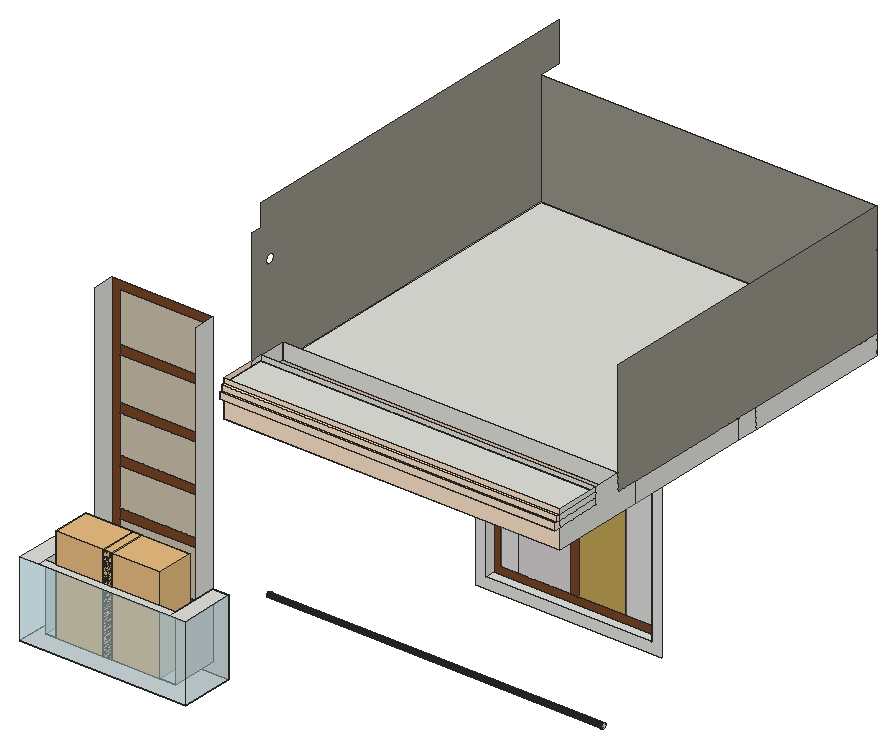
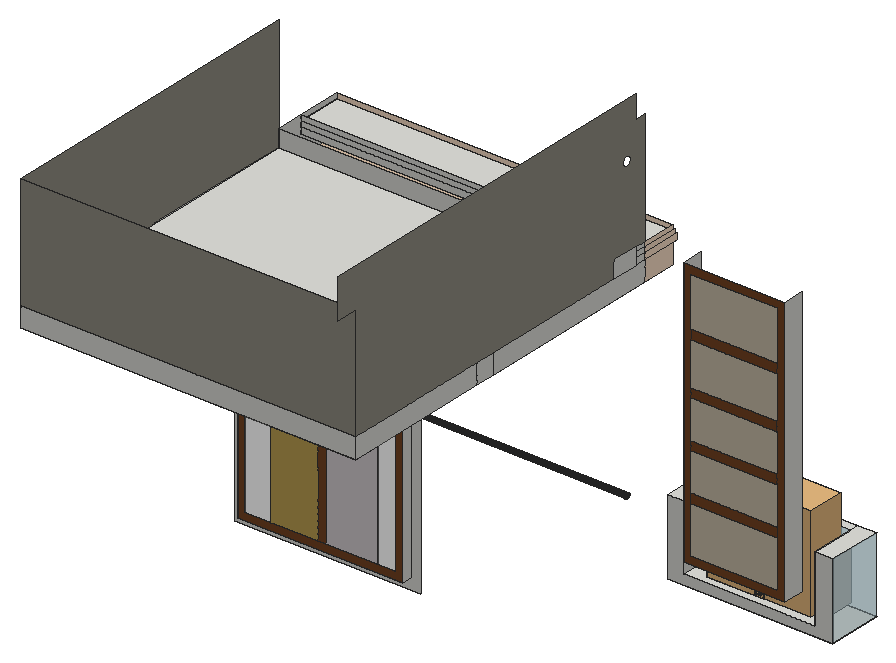
# SketchUp Ruby script. Lengths in inches.
U = 1.inch
M = Sketchup.active_model
def pt(a) = Geom::Point3d.new(a.map { |v| v * U })
def face(e, loops, mat)
  f = e.add_face(loops[0].map { |a| pt(a) })
  loops[1..].each { |l| e.add_face(l.map { |a| pt(a) }).erase! }
  f.material = f.back_material = mat if mat
  f
end
# faces: each face lists its corners as indices into pts; further lists are holes
def faces(e, pts, list, mat = nil) = list.each { |f| face(e, (f[0].is_a?(Array) ? f : [f]).map { |l| l.map { |i| pts[i] } }, mat) }
# xy, xz, yz: faces in a plane at the given z, y or x. An outline is a flat list of corners, or four numbers for a rectangle; further outlines are holes
def ring(l) = l.size == 4 ? [[l[0], l[1]], [l[2], l[1]], [l[2], l[3]], [l[0], l[3]]] : l.each_slice(2).to_a
def flat(e, list, mat, &to3) = list.each { |f| face(e, (f[0].is_a?(Array) ? f : [f]).map { |l| ring(l).map { |u, v| to3.(u, v) } }, mat) }
def xy(e, z, list, mat = nil) = flat(e, list, mat) { |x, y| [x, y, z] }
def xz(e, y, list, mat = nil) = flat(e, list, mat) { |x, z| [x, y, z] }
def yz(e, x, list, mat = nil) = flat(e, list, mat) { |y, z| [x, y, z] }
def lines(e, pts, list) = list.each { |a, b| e.add_line(pt(pts[a]), pt(pts[b])) }
# prism: a flat outline (further loops are holes) pulled along v
def prism(e, loops, v, mat = nil)
  f = face(e, loops, mat); d = Geom::Vector3d.new(v.map { |x| x * U })
  f.pushpull(f.normal.samedirection?(d) ? d.length : -d.length)
end
def box(e, o, s, mat = nil) = prism(e, [[o, [o[0] + s[0], o[1], o[2]], [o[0] + s[0], o[1] + s[1], o[2]], [o[0], o[1] + s[1], o[2]]]], [0, 0, s[2]], mat)
def at(x, y, z, deg = 0) = Geom::Transformation.translation(pt([x, y, z])) * Geom::Transformation.rotation(ORIGIN, Z_AXIS, deg.degrees)
def axes(o, x, y, z) = Geom::Transformation.new([*x, 0, *y, 0, *z, 0, *pt(o).to_a, 1])
def part(name) = M.definitions.add(name)
# library, detail: a bought-in or finely detailed component or shape, given as its bounding box
def library(name, o, s) = part(name).tap { |d| box(d.entities, o, s) }
def detail(e, o, s) = box(e.add_group.entities, o, s)
def put(e, d, t, mat = nil) = e.add_instance(d, t).tap { |i| i.material = mat if mat }
def group(e, t, mat = nil) = e.add_group.tap { |g| g.transformation = t; g.material = mat if mat }.entities
root = M.entities
M.materials.add("[Blinds Cellular White]1").color = [217, 211, 213]
M.materials.add("[Blinds Cloth Horizontal]").color = [192, 163, 85]
M.materials.add("[Color C01]").color = [255, 229, 204]
M.materials.add("[Formica Graystone]").color = [149, 146, 135]
M.materials.add("[Formica Laminate Dark]").color = [50, 53, 60]
M.materials.add("[Formica Laminate Light]").color = [213, 189, 164]
M.materials.add("[Siding Rusty Metal]").color = [206, 195, 174]
M.materials.add("[Translucent Glass Gray]").color = [128, 128, 128]
M.materials["[Translucent Glass Gray]"].alpha = 0.5
M.materials.add("[Translucent Glass Safety]").color = [204, 235, 244]
M.materials["[Translucent Glass Safety]"].alpha = 0.5
M.materials.add("[Wood Veneer 01]").color = [120, 70, 37]
c1 = library("Flora+17",[-57.52,158.6,-38.64],[66.99,62.88,77.28])
xy(root,1210.6875,[[114.55,552.4,668.12,733.78]])
xy(root,1243.125,[[176.52,580.17,613.71,733.78]])
xy(root,1330.35,[[218.87,733.78,559.3,805.03]])
xy(root,1365.38,[[1023.52,1367.21,1578.7,1398.39]])
xy(root,1460,[[1548.73,797.03,1550.53,797.27,1552.2,797.96,1553.64,799.06,1554.74,800.5,1555.43,802.17,1555.67,803.97,1555.43,805.77,1554.74,807.4375,1553.64,808.875,1552.2,809.98,1550.53,810.67,1548.73,810.91,1546.9375,810.67,1545.26,809.98,1543.83,808.875,1542.73,807.4375,1542.03,805.77,1541.8,803.97,1542.03,802.17,1542.73,800.5,1543.83,799.06,1545.26,797.96,1546.9375,797.27]])
xy(root,1460.3125,[[1828.92,797.03,1830.72,797.27,1832.39,797.96,1833.83,799.06,1834.93,800.5,1835.62,802.17,1835.86,803.97,1835.62,805.77,1834.93,807.4375,1833.83,808.875,1832.39,809.98,1830.72,810.67,1828.92,810.91,1827.125,810.67,1825.45,809.98,1824.02,808.875,1822.91,807.4375,1822.22,805.77,1821.98,803.97,1822.22,802.17,1822.91,800.5,1824.02,799.06,1825.45,797.96,1827.125,797.27]])
xy(root,1460.71,[[831.73,797.03,833.53,797.27,835.2,797.96,836.64,799.06,837.74,800.5,838.43,802.17,838.67,803.97,838.43,805.77,837.74,807.4375,836.64,808.875,835.2,809.98,833.53,810.67,832.41,810.82,831.05,810.82,829.9375,810.67,828.26,809.98,826.83,808.875,825.73,807.4375,825.03,805.77,824.8,803.97,825.03,802.17,825.73,800.5,826.83,799.06,828.26,797.96,829.9375,797.27],[831.05,810.82,832.41,810.82,831.73,810.91]])
xy(root,1460.9375,[[1269.3,797.03,1271.09,797.27,1272.76,797.96,1274.2,799.06,1275.3,800.5,1276,802.17,1276.23,803.97,1276,805.77,1275.3,807.4375,1274.2,808.875,1272.76,809.98,1271.09,810.67,1269.3,810.91,1267.5,810.67,1265.83,809.98,1264.39,808.875,1263.29,807.4375,1262.59,805.77,1262.36,803.97,1262.59,802.17,1263.29,800.5,1264.39,799.06,1265.83,797.96,1267.5,797.27]])
xy(root,1462.7,[[778.8,797.03,780.59,797.27,782.26,797.96,783.7,799.06,784.8,800.5,785.5,802.17,785.73,803.97,785.5,805.77,784.8,807.4375,783.7,808.875,782.26,809.98,780.59,810.67,778.8,810.91,777,810.67,775.33,809.98,773.89,808.875,772.79,807.4375,772.09,805.77,771.86,803.97,772.09,802.17,772.79,800.5,773.89,799.06,775.33,797.96,777,797.27],[893.3,797.03,895.09,797.27,896.76,797.96,898.2,799.06,899.3,800.5,900,802.17,900.23,803.97,900,805.77,899.3,807.4375,898.2,808.875,896.76,809.98,895.09,810.67,893.3,810.91,891.5,810.67,889.83,809.98,888.39,808.875,887.29,807.4375,886.59,805.77,886.36,803.97,886.59,802.17,887.29,800.5,888.39,799.06,889.83,797.96,891.5,797.27],[959.23,797.03,961.03,797.27,962.7,797.96,964.14,799.06,965.24,800.5,965.93,802.17,966.17,803.97,965.93,805.77,965.24,807.4375,964.14,808.875,962.7,809.98,961.03,810.67,959.23,810.91,957.4375,810.67,955.76,809.98,954.33,808.875,953.23,807.4375,952.53,805.77,952.3,803.97,952.53,802.17,953.23,800.5,954.33,799.06,955.76,797.96,957.4375,797.27],[1015.98,797.03,1017.78,797.27,1019.45,797.96,1020.89,799.06,1021.99,800.5,1022.68,802.17,1022.92,803.97,1022.68,805.77,1021.99,807.4375,1020.89,808.875,1019.45,809.98,1017.78,810.67,1015.98,810.91,1014.1875,810.67,1012.51,809.98,1011.08,808.875,1009.98,807.4375,1009.28,805.77,1009.05,803.97,1009.28,802.17,1009.98,800.5,1011.08,799.06,1012.51,797.96,1014.1875,797.27],[1072.61,797.03,1074.4,797.27,1076.08,797.96,1077.51,799.06,1078.62,800.5,1079.31,802.17,1079.55,803.97,1079.31,805.77,1078.62,807.4375,1077.51,808.875,1076.08,809.98,1074.4,810.67,1072.61,810.91,1070.8125,810.67,1069.14,809.98,1067.7,808.875,1066.6,807.4375,1065.91,805.77,1065.67,803.97,1065.91,802.17,1066.6,800.5,1067.7,799.06,1069.14,797.96,1070.8125,797.27],
  [1665.86,797.03,1667.65,797.27,1669.33,797.96,1670.76,799.06,1671.87,800.5,1672.56,802.17,1672.8,803.97,1672.56,805.77,1671.87,807.4375,1670.76,808.875,1669.33,809.98,1667.65,810.67,1665.86,810.91,1664.0625,810.67,1662.39,809.98,1660.95,808.875,1659.85,807.4375,1659.16,805.77,1658.92,803.97,1659.16,802.17,1659.85,800.5,1660.95,799.06,1662.39,797.96,1664.0625,797.27],[1721.48,797.03,1723.28,797.27,1724.95,797.96,1726.39,799.06,1727.49,800.5,1728.18,802.17,1728.42,803.97,1728.18,805.77,1727.49,807.4375,1726.39,808.875,1724.95,809.98,1723.28,810.67,1721.48,810.91,1719.6875,810.67,1718.01,809.98,1716.58,808.875,1715.48,807.4375,1714.78,805.77,1714.55,803.97,1714.78,802.17,1715.48,800.5,1716.58,799.06,1718.01,797.96,1719.6875,797.27],[1772.17,797.03,1773.97,797.27,1775.64,797.96,1777.08,799.06,1778.18,800.5,1778.87,802.17,1779.11,803.97,1778.87,805.77,1778.18,807.4375,1777.08,808.875,1775.64,809.98,1773.97,810.67,1772.17,810.91,1770.375,810.67,1768.7,809.98,1767.27,808.875,1766.16,807.4375,1765.47,805.77,1765.23,803.97,1765.47,802.17,1766.16,800.5,1767.27,799.06,1768.7,797.96,1770.375,797.27]])
xy(root,1463.4375,[[114.55,552.4,176.52,733.78],[176.52,552.4,613.71,580.17],[613.71,552.4,668.12,733.78]])
xy(root,1464.6875,[[1135.17,797.03,1136.97,797.27,1138.64,797.96,1140.08,799.06,1141.18,800.5,1141.87,802.17,1142.11,803.97,1141.87,805.77,1141.18,807.4375,1140.08,808.875,1138.64,809.98,1136.97,810.67,1135.85,810.82,1134.49,810.82,1133.375,810.67,1131.7,809.98,1130.27,808.875,1129.16,807.4375,1128.47,805.77,1128.23,803.97,1128.47,802.17,1129.16,800.5,1130.27,799.06,1131.7,797.96,1133.375,797.27],[1205.55,797.03,1207.34,797.27,1209.01,797.96,1210.45,799.06,1211.55,800.5,1212.25,802.17,1212.48,803.97,1212.25,805.77,1211.55,807.4375,1210.45,808.875,1209.01,809.98,1207.34,810.67,1206.23,810.82,1204.87,810.82,1203.75,810.67,1202.08,809.98,1200.64,808.875,1199.54,807.4375,1198.84,805.77,1198.61,803.97,1198.84,802.17,1199.54,800.5,1200.64,799.06,1202.08,797.96,1203.75,797.27],[1326.55,797.03,1328.34,797.27,1330.01,797.96,1331.45,799.06,1332.55,800.5,1333.25,802.17,1333.48,803.97,1333.25,805.77,1332.55,807.4375,1331.45,808.875,1330.01,809.98,1328.34,810.67,1327.23,810.82,1325.87,810.82,1324.75,810.67,1323.08,809.98,1321.64,808.875,1320.54,807.4375,1319.84,805.77,1319.61,803.97,1319.84,802.17,1320.54,800.5,1321.64,799.06,1323.08,797.96,1324.75,797.27],[1386.05,797.03,1387.84,797.27,1389.51,797.96,1390.95,799.06,1392.05,800.5,1392.75,802.17,1392.98,803.97,1392.75,805.77,1392.05,807.4375,1390.95,808.875,1389.51,809.98,1387.84,810.67,1386.73,810.82,1385.37,810.82,1384.25,810.67,1382.58,809.98,1381.14,808.875,1380.04,807.4375,1379.34,805.77,1379.11,803.97,1379.34,802.17,1380.04,800.5,1381.14,799.06,1382.58,797.96,1384.25,797.27],[1435.55,797.03,1437.34,797.27,1439.01,797.96,1440.45,799.06,1441.55,800.5,1442.25,802.17,1442.48,803.97,1442.25,805.77,1441.55,807.4375,1440.45,808.875,1439.01,809.98,1437.34,810.67,1436.23,810.82,1434.87,810.82,1433.75,810.67,1432.08,809.98,1430.64,808.875,1429.54,807.4375,1428.84,805.77,1428.61,803.97,1428.84,802.17,1429.54,800.5,1430.64,799.06,1432.08,797.96,1433.75,797.27],
  [1608.3,797.03,1610.09,797.27,1611.76,797.96,1613.2,799.06,1614.3,800.5,1615,802.17,1615.23,803.97,1615,805.77,1614.3,807.4375,1613.2,808.875,1611.76,809.98,1610.09,810.67,1608.98,810.82,1607.62,810.82,1606.5,810.67,1604.83,809.98,1603.39,808.875,1602.29,807.4375,1601.59,805.77,1601.36,803.97,1601.59,802.17,1602.29,800.5,1603.39,799.06,1604.83,797.96,1606.5,797.27],[1134.49,810.82,1135.85,810.82,1135.17,810.91],[1204.87,810.82,1206.23,810.82,1205.55,810.91],[1325.87,810.82,1327.23,810.82,1326.55,810.91],[1385.37,810.82,1386.73,810.82,1386.05,810.91],
  [1434.87,810.82,1436.23,810.82,1435.55,810.91],[1607.62,810.82,1608.98,810.82,1608.3,810.91]])
xy(root,1466.5,[[1489.3,797.03,1491.09,797.27,1492.76,797.96,1494.2,799.06,1495.3,800.5,1496,802.17,1496.23,803.97,1496,805.77,1495.3,807.4375,1494.2,808.875,1492.76,809.98,1491.09,810.67,1489.3,810.91,1487.5,810.67,1485.83,809.98,1484.39,808.875,1483.29,807.4375,1482.59,805.77,1482.36,803.97,1482.59,802.17,1483.29,800.5,1484.39,799.06,1485.83,797.96,1487.5,797.27]])
xy(root,1920.56,[[1023.52,1367.21,1578.7,1398.39]])
xy(root,2073.3125,[[911.88,741.63,899.73,743.23,888.41,747.92,878.69,755.38,871.23,765.1,866.54,776.42,864.94,788.57,866.54,800.72,871.23,812.04,878.69,821.76,888.41,829.22,899.73,833.91,911.88,835.5,924.03,833.91,935.35,829.22,945.07,821.76,952.53,812.04,957.22,800.72,958.82,788.57,957.22,776.42,952.53,765.1,945.07,755.38,935.35,747.92,924.03,743.23],[1252.07,741.63,1239.92,743.23,1228.6,747.92,1218.88,755.38,1211.42,765.1,1206.73,776.42,1205.13,788.57,1206.73,800.72,1211.42,812.04,1218.88,821.76,1228.6,829.22,1239.92,833.91,1252.07,835.5,1264.22,833.91,1275.54,829.22,1285.26,821.76,1292.72,812.04,1297.41,800.72,1299.01,788.57,1297.41,776.42,1292.72,765.1,1285.26,755.38,1275.54,747.92,1264.22,743.23],[1632.32,741.63,1620.17,743.23,1608.85,747.92,1599.13,755.38,1591.67,765.1,1586.98,776.42,1585.38,788.57,1586.98,800.72,1591.67,812.04,1599.13,821.76,1608.85,829.22,1620.17,833.91,1632.32,835.5,1644.47,833.91,1655.79,829.22,1665.51,821.76,1672.97,812.04,1677.66,800.72,1679.26,788.57,1677.66,776.42,1672.97,765.1,1665.51,755.38,1655.79,747.92,1644.47,743.23],[746.18,1367.21,1870.17,1437.7],[746.18,1437.7,1870.17,1944.66]])
xy(root,2073.3125,[[[746.18,617.28,1870.17,1367.21],[911.88,741.63,924.03,743.23,935.35,747.92,945.07,755.38,952.53,765.1,957.22,776.42,958.82,788.57,957.22,800.72,952.53,812.04,945.07,821.76,935.35,829.22,924.03,833.91,911.88,835.5,899.73,833.91,888.41,829.22,878.69,821.76,871.23,812.04,866.54,800.72,864.94,788.57,866.54,776.42,871.23,765.1,878.69,755.38,888.41,747.92,899.73,743.23],[1632.32,741.63,1644.47,743.23,1655.79,747.92,1665.51,755.38,1672.97,765.1,1677.66,776.42,1679.26,788.57,1677.66,800.72,1672.97,812.04,1665.51,821.76,1655.79,829.22,1644.47,833.91,1632.32,835.5,1620.17,833.91,1608.85,829.22,1599.13,821.76,1591.67,812.04,1586.98,800.72,1585.38,788.57,1586.98,776.42,1591.67,765.1,1599.13,755.38,1608.85,747.92,1620.17,743.23],[1252.07,741.63,1264.22,743.23,1275.54,747.92,1285.26,755.38,1292.72,765.1,1297.41,776.42,1299.01,788.57,1297.41,800.72,1292.72,812.04,1285.26,821.76,1275.54,829.22,1264.22,833.91,1252.07,835.5,1239.92,833.91,1228.6,829.22,1218.88,821.76,1211.42,812.04,1206.73,800.72,1205.13,788.57,1206.73,776.42,1211.42,765.1,1218.88,755.38,1228.6,747.92,1239.92,743.23]]],"[Formica Laminate Light]")
xy(root,2140.0625,[[746.18,617.28,1870.17,769.97],[746.18,862.78,1870.17,1944.66]])
xy(root,2140.0625,[[746.18,597.72,1870.17,617.28]],"[Color C01]")
xy(root,2161.6875,[[746.18,606.84,1870.17,769.97]])
xy(root,2161.6875,[[746.18,597.72,1870.17,606.84]],"[Color C01]")
xy(root,2179.375,[[746.18,617.28,1870.17,769.97]])
xy(root,2179.375,[[746.18,606.84,1870.17,617.28]],"[Color C01]")
xz(root,552.4,[[114.55,1210.6875,668.12,1463.4375]],"[Translucent Glass Safety]")
xz(root,580.17,[[176.52,1243.125,613.71,1463.4375]],"[Translucent Glass Safety]")
xz(root,597.72,[[746.18,2140.0625,1870.17,2161.6875]],"[Color C01]")
xz(root,606.84,[[746.18,2161.6875,1870.17,2179.375]],"[Color C01]")
xz(root,617.28,[[746.18,2073.3125,1870.17,2140.0625],[746.18,2179.375,1870.17,2196.1875]],"[Color C01]")
xz(root,733.78,[[114.55,1210.6875,114.55,1463.4375,176.52,1463.4375,176.52,1243.125,613.71,1243.125,613.71,1463.4375,668.12,1463.4375,668.12,1210.6875]])
xz(root,769.97,[[746.18,2140.0625,1870.17,2161.6875],[746.18,2161.6875,1870.17,2179.375],[746.18,2179.375,1870.17,2196.1875]])
xz(root,805.03,[[245.45,1356.94,532.72,1514.27],[245.45,1546.53,532.72,1672.71],[245.45,1704.97,532.72,1831.9],[245.45,1864.16,532.72,2006.21],[245.45,2038.47,532.72,2202.76]],"[Siding Rusty Metal]")
xz(root,805.03,[[[218.87,1330.35,559.3,2229.35],[245.45,1356.94,532.72,2202.76]],[245.45,1514.27,532.72,1546.53],[245.45,1672.71,532.72,1704.97],[245.45,1831.9,532.72,1864.16],[245.45,2006.21,532.72,2038.47]],"[Wood Veneer 01]")
xz(root,862.78,[[746.18,2140.0625,1870.17,2196.1875]])
xz(root,1367.21,[[[988.74,1330.6,1613.49,1955.35],[1023.52,1365.38,1578.7,1920.56]]])
xz(root,1398.39,[[1108.38,1390.59,1282.22,1895.36]],"[Blinds Cellular White]1")
xz(root,1398.39,[[1311.1,1390.59,1466.57,1895.36]],"[Blinds Cloth Horizontal]")
xz(root,1398.39,[[1048.72,1390.59,1108.38,1895.36],[1466.57,1390.59,1553.5,1895.36]],"[Translucent Glass Gray]")
xz(root,1398.39,[[[1023.52,1365.38,1578.7,1920.56],[1048.72,1390.59,1553.5,1895.36]],[1282.22,1390.59,1311.1,1895.36]],"[Wood Veneer 01]")
xz(root,1944.66,[[746.18,2073.3125,1870.17,2140.0625]])
xz(root,1944.66,[[746.18,2140.0625,1870.17,2522.1875]],"[Formica Graystone]")
yz(root,114.55,[[552.4,1210.6875,733.78,1463.4375]],"[Translucent Glass Safety]")
yz(root,176.52,[[580.17,1243.125,733.78,1463.4375]])
yz(root,218.87,[[733.78,1330.35,805.03,2229.35]])
yz(root,559.3,[[733.78,1330.35,805.03,2229.35]])
yz(root,613.71,[[580.17,1243.125,733.78,1463.4375]])
yz(root,668.12,[[552.4,1210.6875,733.78,1463.4375]],"[Translucent Glass Safety]")
yz(root,746.18,[[733.78,2073.3125,1367.21,2140.0625],[1367.21,2073.3125,1437.7,2140.0625],[1437.7,2073.3125,1944.66,2140.0625],[733.78,2140.0625,769.97,2161.6875],[769.97,2140.0625,862.78,2196.1875],
  [733.78,2161.6875,769.97,2179.375],[733.78,2179.375,769.97,2196.1875]])
yz(root,746.18,[[617.28,2073.3125,733.78,2140.0625],[597.72,2140.0625,733.78,2161.6875],[606.84,2161.6875,733.78,2179.375],[617.28,2179.375,733.78,2196.1875]],"[Color C01]")
yz(root,746.18,[[[862.78,2140.0625,1944.66,2140.0625,1944.66,2522.1875,2018.8,2522.1875,2018.8,2654.3125,769.97,2654.3125,769.97,2578.28,733.78,2578.28,733.78,2196.1875,862.78,2196.1875],[808.34,2453.16,804.29,2453.6875,800.53,2455.25,797.29,2457.73,794.81,2460.97,793.25,2464.74,792.71,2468.78,793.25,2472.82,794.81,2476.59,797.29,2479.83,800.53,2482.3125,804.29,2483.875,808.34,2484.41,812.38,2483.875,816.15,2482.3125,819.39,2479.83,821.87,2476.59,823.43,2472.82,823.96,2468.78,823.43,2464.74,821.87,2460.97,819.39,2457.73,816.15,2455.25,812.38,2453.6875]]],"[Formica Graystone]")
yz(root,1023.52,[[1367.21,1365.38,1398.39,1920.56]])
yz(root,1578.7,[[1367.21,1365.38,1398.39,1920.56]])
yz(root,1870.17,[[803.39,1455.01,805.38,1455.27,807.24,1456.04,808.83,1457.26,810.05,1458.85,810.82,1460.71,811.08,1462.7,810.82,1464.6875,810.05,1466.54,808.83,1468.13,807.24,1469.35,805.38,1470.12,803.39,1470.38,801.4,1470.12,799.55,1469.35,797.96,1468.13,796.73,1466.54,795.97,1464.6875,795.71,1462.7,795.97,1460.71,796.73,1458.85,797.96,1457.26,799.55,1456.04,801.4,1455.27],[617.28,2073.3125,930.73,2073.3125,930.73,2140.0625,862.78,2140.0625,862.78,2196.1875,769.97,2196.1875,769.97,2140.0625,617.28,2140.0625],[930.73,2073.3125,1367.21,2140.0625],[1367.21,2073.3125,1437.7,2140.0625],[1437.7,2073.3125,1944.66,2140.0625],
  [617.28,2140.0625,769.97,2161.6875],[617.28,2161.6875,769.97,2179.375],[617.28,2179.375,769.97,2196.1875]])
yz(root,1870.17,[[597.72,2140.0625,617.28,2161.6875],[606.84,2161.6875,617.28,2179.375]],"[Color C01]")
yz(root,1870.17,[[862.78,2140.0625,1944.66,2522.1875]],"[Formica Graystone]")
p = [[1870.17,803.39,1455.01],[1870.17,801.4,1455.27],[746.18,801.4,1455.27],[746.18,803.39,1455.01],[1870.17,805.38,1455.27],[746.18,805.38,1455.27],
  [1870.17,799.55,1456.04],[746.18,799.55,1456.04],[1870.17,807.24,1456.04],[746.18,807.24,1456.04],[1870.17,797.96,1457.26],[746.18,797.96,1457.26],
  [1870.17,808.83,1457.26],[746.18,808.83,1457.26],[1870.17,796.73,1458.85],[746.18,796.73,1458.85],[1870.17,810.05,1458.85],[746.18,810.05,1458.85],
  [1870.17,795.97,1460.71],[746.18,795.97,1460.71],[1870.17,810.82,1460.71],[746.18,810.82,1460.71],[831.05,810.82,1460.71],[832.41,810.82,1460.71],
  [1870.17,795.71,1462.7],[746.18,795.71,1462.7],[1870.17,811.08,1462.7],[746.18,811.08,1462.7],[1870.17,795.97,1464.6875],[746.18,795.97,1464.6875],
  [1870.17,810.82,1464.6875],[746.18,810.82,1464.6875],[1134.49,810.82,1464.6875],[1135.85,810.82,1464.6875],[1204.87,810.82,1464.6875],[1206.23,810.82,1464.6875],
  [1325.87,810.82,1464.6875],[1327.23,810.82,1464.6875],[1385.37,810.82,1464.6875],[1386.73,810.82,1464.6875],[1434.87,810.82,1464.6875],[1436.23,810.82,1464.6875],
  [1607.62,810.82,1464.6875],[1608.98,810.82,1464.6875],[1870.17,796.73,1466.54],[746.18,796.73,1466.54],[1870.17,810.05,1466.54],[746.18,810.05,1466.54],
  [1870.17,797.96,1468.13],[746.18,797.96,1468.13],[1870.17,808.83,1468.13],[746.18,808.83,1468.13],[1870.17,799.55,1469.35],[746.18,799.55,1469.35],
  [1870.17,807.24,1469.35],[746.18,807.24,1469.35],[1870.17,801.4,1470.12],[746.18,801.4,1470.12],[1870.17,805.38,1470.12],[746.18,805.38,1470.12],
  [1870.17,803.39,1470.38],[746.18,803.39,1470.38]]
faces(root,p,[[0,1,2,3],[4,0,3,5],[1,6,7,2],[8,4,5,9],[6,10,11,7],[12,8,9,13],[10,14,15,11],[16,12,13,17],
  [14,18,19,15],[20,16,17,21,22,23],[18,24,25,19],[26,20,23,22,21,27],[24,28,29,25],[30,26,27,31,32,33,34,35,36,37,38,39,40,41,42,43],[28,44,45,29],[46,30,43,42,41,40,39,38,37,36,35,34,33,32,31,47],
  [44,48,49,45],[50,46,47,51],[48,52,53,49],[54,50,51,55],[52,56,57,53],[58,54,55,59],[56,60,61,57],[60,58,59,61]],"[Formica Laminate Dark]")
put(root,c1,axes([372.83,262.72,1402.87],[2.8238,0,0],[0,2,0],[0,0,4.134]))
put(root,c1,axes([532.14,262.72,1402.87],[2.8238,0,0],[0,2,0],[0,0,4.134]))
